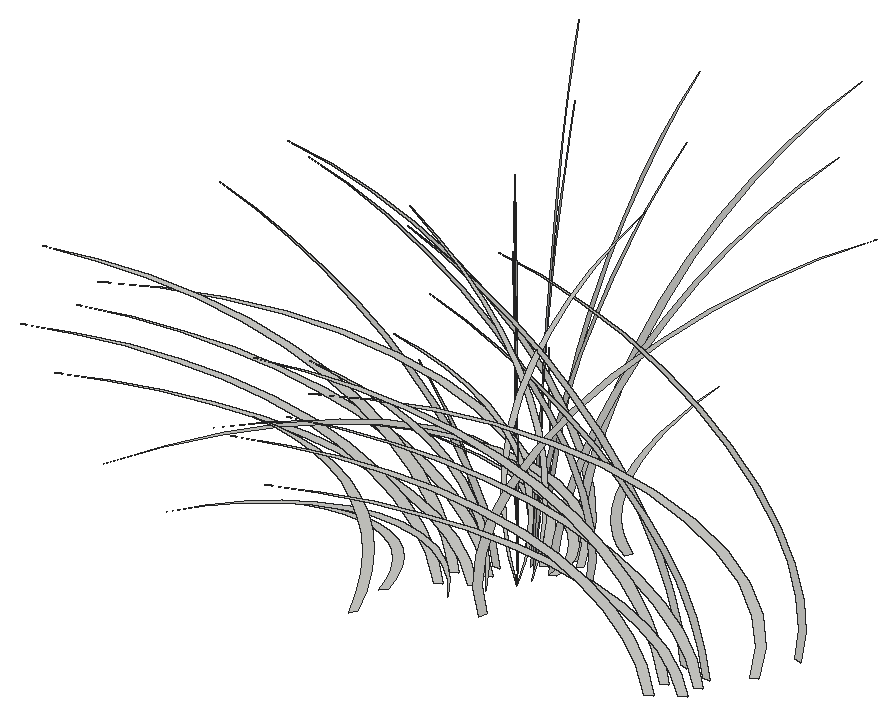
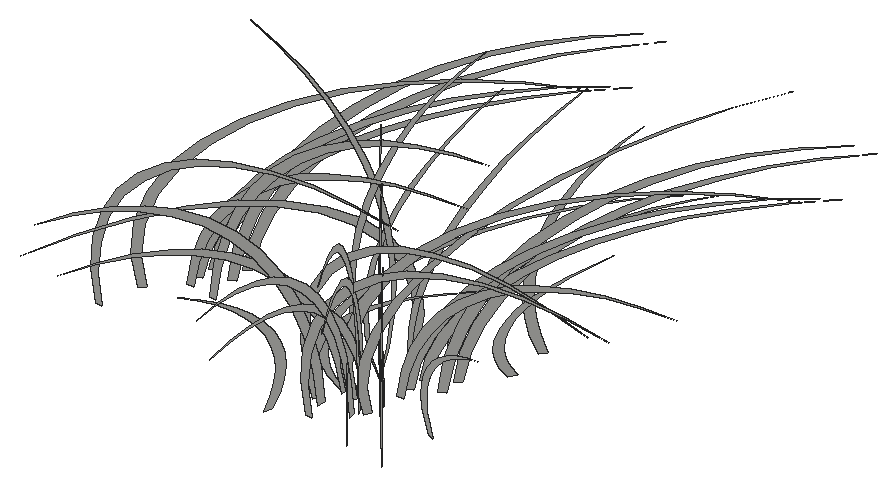
# SketchUp Ruby script. Lengths in inches.
U = 1.inch
M = Sketchup.active_model
def pt(a) = Geom::Point3d.new(a.map { |v| v * U })
def face(e, loops, mat)
  f = e.add_face(loops[0].map { |a| pt(a) })
  loops[1..].each { |l| e.add_face(l.map { |a| pt(a) }).erase! }
  f.material = f.back_material = mat if mat
  f
end
# faces: each face lists its corners as indices into pts; further lists are holes
def faces(e, pts, list, mat = nil) = list.each { |f| face(e, (f[0].is_a?(Array) ? f : [f]).map { |l| l.map { |i| pts[i] } }, mat) }
# xy, xz, yz: faces in a plane at the given z, y or x. An outline is a flat list of corners, or four numbers for a rectangle; further outlines are holes
def ring(l) = l.size == 4 ? [[l[0], l[1]], [l[2], l[1]], [l[2], l[3]], [l[0], l[3]]] : l.each_slice(2).to_a
def flat(e, list, mat, &to3) = list.each { |f| face(e, (f[0].is_a?(Array) ? f : [f]).map { |l| ring(l).map { |u, v| to3.(u, v) } }, mat) }
def xy(e, z, list, mat = nil) = flat(e, list, mat) { |x, y| [x, y, z] }
def xz(e, y, list, mat = nil) = flat(e, list, mat) { |x, z| [x, y, z] }
def yz(e, x, list, mat = nil) = flat(e, list, mat) { |y, z| [x, y, z] }
def lines(e, pts, list) = list.each { |a, b| e.add_line(pt(pts[a]), pt(pts[b])) }
# prism: a flat outline (further loops are holes) pulled along v
def prism(e, loops, v, mat = nil)
  f = face(e, loops, mat); d = Geom::Vector3d.new(v.map { |x| x * U })
  f.pushpull(f.normal.samedirection?(d) ? d.length : -d.length)
end
def box(e, o, s, mat = nil) = prism(e, [[o, [o[0] + s[0], o[1], o[2]], [o[0] + s[0], o[1] + s[1], o[2]], [o[0], o[1] + s[1], o[2]]]], [0, 0, s[2]], mat)
def at(x, y, z, deg = 0) = Geom::Transformation.translation(pt([x, y, z])) * Geom::Transformation.rotation(ORIGIN, Z_AXIS, deg.degrees)
def axes(o, x, y, z) = Geom::Transformation.new([*x, 0, *y, 0, *z, 0, *pt(o).to_a, 1])
def part(name) = M.definitions.add(name)
# library, detail: a bought-in or finely detailed component or shape, given as its bounding box
def library(name, o, s) = part(name).tap { |d| box(d.entities, o, s) }
def detail(e, o, s) = box(e.add_group.entities, o, s)
def put(e, d, t, mat = nil) = e.add_instance(d, t).tap { |i| i.material = mat if mat }
def group(e, t, mat = nil) = e.add_group.tap { |g| g.transformation = t; g.material = mat if mat }.entities
root = M.entities
p = [[75.43,134.13,1.9375],[799.67,134.13,1.9375]]
lines(root,p,[[0,1]])
g1 = group(root,at(436.95,262.29,0))
p = [[-18.45,-9.5625,18.05],[-21.23,-11,18.53],[-18.53,-9.61,17.95],[-15.93,-8.26,17.15],[-13.45,-6.97,16.14],[-11.12,-5.76,14.93],
  [-8.96,-4.64,13.53],[-7,-3.63,11.96],[-5.26,-2.73,10.23],[-3.77,-1.95,8.37],[-2.53,-1.3125,6.39],[-1.5625,-0.81,4.32],
  [-0.875,-0.45,2.18],[-0.48,-0.25,0],[0,0,0],[-0.32,-0.17,2.23],[-0.97,-0.5,4.43],[-1.92,-0.99,6.55],
  [-3.16,-1.64,8.57],[-4.69,-2.43,10.47],[-6.48,-3.36,12.22],[-8.51,-4.41,13.8],[-10.75,-5.57,15.1875],[-13.17,-6.83,16.37],
  [-15.75,-8.16,17.33]]
faces(g1,p,[[0,1,2,3,4,5,6,7,8,9,10,11,12,13,14,15,16,17,18,19,20,21,22,23,24]])
g2 = group(root,at(438.46,264.06,0))
p = [[-20.46,3.64,14.56],[-23.54,4.19,14.94],[-20.55,3.66,14.48],[-17.67,3.15,13.83],[-14.91,2.66,13.02],[-12.33,2.2,12.04],
  [-9.93,1.77,10.91],[-7.76,1.38,9.64],[-5.84,1.04,8.25],[-4.18,0.74,6.75],[-2.8,0.5,5.15],[-1.73,0.31,3.49],
  [-0.97,0.17,1.76],[-0.53,0.09,0],[0,0,0],[-0.36,0.0625,1.8],[-1.07,0.19,3.57],[-2.125,0.38,5.28],
  [-3.51,0.625,6.91],[-5.2,0.93,8.44],[-7.1875,1.28,9.85],[-9.43,1.68,11.13],[-11.92,2.125,12.25],[-14.61,2.6,13.2],
  [-17.46,3.11,13.97]]
faces(g2,p,[[0,1,2,3,4,5,6,7,8,9,10,11,12,13,14,15,16,17,18,19,20,21,22,23,24]])
g3 = group(root,at(437,260.8,0))
p = [[-17.17,-11.7,15.34],[-19.76,-13.47,15.75],[-17.25,-11.76,15.26],[-14.83,-10.11,14.58],[-12.52,-8.53,13.72],[-10.35,-7.05,12.69],
  [-8.34,-5.68,11.5],[-6.52,-4.44,10.16],[-4.9,-3.34,8.7],[-3.51,-2.39,7.11],[-2.35,-1.6,5.43],[-1.45,-0.99,3.67],
  [-0.82,-0.56,1.86],[-0.45,-0.3,0],[0,0,0],[-0.3,-0.21,1.9],[-0.9,-0.61,3.76],[-1.78,-1.22,5.57],
  [-2.95,-2.01,7.28],[-4.37,-2.98,8.9],[-6.03,-4.11,10.39],[-7.92,-5.4,11.73],[-10,-6.82,12.91],[-12.26,-8.36,13.91],
  [-14.66,-9.99,14.73]]
faces(g3,p,[[0,1,2,3,4,5,6,7,8,9,10,11,12,13,14,15,16,17,18,19,20,21,22,23,24]])
g4 = group(root,at(438.67,263.18,0))
p = [[-18.45,-9.5625,14.56],[-21.23,-11,14.94],[-18.53,-9.61,14.48],[-15.93,-8.26,13.83],[-13.45,-6.97,13.02],[-11.12,-5.76,12.04],
  [-8.96,-4.64,10.91],[-7,-3.63,9.64],[-5.26,-2.73,8.25],[-3.77,-1.95,6.75],[-2.53,-1.3125,5.15],[-1.5625,-0.81,3.49],
  [-0.875,-0.45,1.76],[-0.48,-0.25,0],[0,0,0],[-0.32,-0.17,1.8],[-0.97,-0.5,3.57],[-1.92,-0.99,5.28],
  [-3.16,-1.64,6.91],[-4.69,-2.43,8.44],[-6.48,-3.36,9.85],[-8.51,-4.41,11.13],[-10.75,-5.57,12.25],[-13.17,-6.83,13.2],
  [-15.75,-8.16,13.97]]
faces(g4,p,[[0,1,2,3,4,5,6,7,8,9,10,11,12,13,14,15,16,17,18,19,20,21,22,23,24]])
g5 = group(root,at(438.67,263.18,0))
p = [[-18.45,-9.5625,14.56],[-21.23,-11,14.94],[-18.53,-9.61,14.48],[-15.93,-8.26,13.83],[-13.45,-6.97,13.02],[-11.12,-5.76,12.04],
  [-8.96,-4.64,10.91],[-7,-3.63,9.64],[-5.26,-2.73,8.25],[-3.77,-1.95,6.75],[-2.53,-1.3125,5.15],[-1.5625,-0.81,3.49],
  [-0.875,-0.45,1.76],[-0.48,-0.25,0],[0,0,0],[-0.32,-0.17,1.8],[-0.97,-0.5,3.57],[-1.92,-0.99,5.28],
  [-3.16,-1.64,6.91],[-4.69,-2.43,8.44],[-6.48,-3.36,9.85],[-8.51,-4.41,11.13],[-10.75,-5.57,12.25],[-13.17,-6.83,13.2],
  [-15.75,-8.16,13.97]]
faces(g5,p,[[0,1,2,3,4,5,6,7,8,9,10,11,12,13,14,15,16,17,18,19,20,21,22,23,24]])
g6 = group(root,at(441.53,268.9,0))
p = [[-0.91,0.16,0],[-0.4,0.07,0],[0,0,2.0625],[-0.16,0.03,4.13],[-0.89,0.16,6.16],[-2.17,0.39,8.1],
  [-3.95,0.7,9.91],[-6.21,1.11,11.52],[-8.88,1.58,12.92],[-11.91,2.12,14.05],[-15.2,2.71,14.9],[-18.68,3.33,15.45],
  [-22.27,3.97,15.67],[-25.88,4.61,15.5625],[-22.34,3.98,15.58],[-18.84,3.36,15.29],[-15.45,2.75,14.71],[-12.26,2.18,13.83],
  [-9.34,1.66,12.68],[-6.75,1.2,11.3],[-4.56,0.8125,9.7],[-2.81,0.5,7.9375],[-1.55,0.28,6.04],[-0.8,0.14,4.05],
  [-0.59,0.1,2.02]]
faces(g6,p,[[0,1,2,3,4,5,6,7,8,9,10,11,12,13,14,15,16,17,18,19,20,21,22,23,24]])
g7 = group(root,at(441.53,268.9,0))
p = [[-0.91,0.16,0],[-0.4,0.07,0],[0,0,2.0625],[-0.16,0.03,4.13],[-0.89,0.16,6.16],[-2.17,0.39,8.1],
  [-3.95,0.7,9.91],[-6.21,1.11,11.52],[-8.88,1.58,12.92],[-11.91,2.12,14.05],[-15.2,2.71,14.9],[-18.68,3.33,15.45],
  [-22.27,3.97,15.67],[-25.88,4.61,15.5625],[-22.34,3.98,15.58],[-18.84,3.36,15.29],[-15.45,2.75,14.71],[-12.26,2.18,13.83],
  [-9.34,1.66,12.68],[-6.75,1.2,11.3],[-4.56,0.8125,9.7],[-2.81,0.5,7.9375],[-1.55,0.28,6.04],[-0.8,0.14,4.05],
  [-0.59,0.1,2.02]]
faces(g7,p,[[0,1,2,3,4,5,6,7,8,9,10,11,12,13,14,15,16,17,18,19,20,21,22,23,24]])
g8 = group(root,at(438.59,261.89,0))
p = [[-17.17,-11.7,12.375],[-19.76,-13.47,12.7],[-17.25,-11.76,12.31],[-14.83,-10.11,11.76],[-12.52,-8.53,11.07],[-10.35,-7.05,10.23],
  [-8.34,-5.68,9.27],[-6.52,-4.44,8.2],[-4.9,-3.34,7.01],[-3.51,-2.39,5.74],[-2.35,-1.6,4.38],[-1.45,-0.99,2.96],
  [-0.82,-0.56,1.5],[-0.45,-0.3,0],[0,0,0],[-0.3,-0.21,1.53],[-0.9,-0.61,3.03],[-1.78,-1.22,4.49],
  [-2.95,-2.01,5.875],[-4.37,-2.98,7.18],[-6.03,-4.11,8.375],[-7.92,-5.4,9.46],[-10,-6.82,10.41],[-12.26,-8.36,11.22],
  [-14.66,-9.99,11.88]]
faces(g8,p,[[0,1,2,3,4,5,6,7,8,9,10,11,12,13,14,15,16,17,18,19,20,21,22,23,24]])
g9 = group(root,at(440.79,266.21,0))
p = [[-0.82,-0.43,0],[-0.36,-0.1875,0],[0,0,2.0625],[-0.15,-0.08,4.13],[-0.8,-0.42,6.16],[-1.95,-1.01,8.1],
  [-3.57,-1.85,9.91],[-5.6,-2.9,11.52],[-8.01,-4.15,12.92],[-10.74,-5.57,14.05],[-13.71,-7.1,14.9],[-16.85,-8.73,15.45],
  [-20.09,-10.41,15.67],[-23.34,-12.1,15.5625],[-20.15,-10.44,15.58],[-16.99,-8.81,15.29],[-13.9375,-7.22,14.71],[-11.06,-5.73,13.83],
  [-8.42,-4.37,12.68],[-6.09,-3.16,11.3],[-4.11,-2.13,9.7],[-2.53,-1.3125,7.9375],[-1.4,-0.72,6.04],[-0.72,-0.375,4.05],
  [-0.53,-0.27,2.02]]
faces(g9,p,[[0,1,2,3,4,5,6,7,8,9,10,11,12,13,14,15,16,17,18,19,20,21,22,23,24]])
g10 = group(root,at(444.39,265.34,0))
p = [[-0.95,0.28,0],[-0.42,0.125,0],[0,0,2.01],[-0.17,0.05,4.04],[-0.93,0.27,6.02],[-2.27,0.66,7.92],
  [-4.14,1.21,9.68],[-6.5,1.9,11.26],[-9.3,2.72,12.62],[-12.46,3.64,13.73],[-15.91,4.65,14.5625],[-19.55,5.72,15.09],
  [-23.3125,6.82,15.31],[-27.08,7.92,15.2],[-23.38,6.84,15.22],[-19.72,5.77,14.94],[-16.17,4.73,14.37],[-12.83,3.75,13.51],
  [-9.77,2.86,12.39],[-7.0625,2.07,11.04],[-4.77,1.39,9.48],[-2.94,0.86,7.75],[-1.62,0.47,5.9],[-0.84,0.25,3.96],
  [-0.61,0.18,1.98]]
faces(g10,p,[[0,1,2,3,4,5,6,7,8,9,10,11,12,13,14,15,16,17,18,19,20,21,22,23,24]])
g11 = group(root,at(435.12,266.09,0))
p = [[-6.53,2.99,7.88],[-5.33,2.44,7.38],[-4.26,1.95,6.83],[-3.3,1.51,6.24],[-2.48,1.14,5.62],[-1.81,0.83,4.96],
  [-1.28,0.58,4.27],[-0.9,0.41,3.57],[-0.68,0.31,2.86],[-0.61,0.28,2.13],[-0.71,0.32,1.41],[-0.96,0.4375,0.7],
  [-1.37,0.625,0],[-0.84,0.38,0],[-0.39,0.18,0.71],[-0.11,0.05,1.43],[0,0,2.17],[-0.07,0.03,2.9],
  [-0.32,0.15,3.63],[-0.74,0.34,4.34],[-1.33,0.61,5.03],[-2.08,0.95,5.69],[-2.99,1.37,6.3125],[-4.04,1.85,6.89],
  [-5.22,2.39,7.41]]
faces(g11,p,[[0,1,2,3,4,5,6,7,8,9,10,11,12,13,14,15,16,17,18,19,20,21,22,23,24]])
g12 = group(root,at(437.88,266.32,0))
p = [[-10.66,12.98,9.9],[-9.23,11.23,9.83],[-7.82,9.52,9.59],[-6.46,7.86,9.18],[-5.18,6.3,8.61],[-3.99,4.86,7.88],
  [-2.93,3.57,7.02],[-2.02,2.46,6.03],[-1.27,1.54,4.95],[-0.6875,0.84,3.78],[-0.29,0.36,2.55],[-0.1,0.12,1.28],
  [-0.09,0.12,0],[0,0,1.3],[-0.125,0.15,2.61],[-0.47,0.57,3.875],[-1.02,1.24,5.09],[-1.77,2.15,6.21],
  [-2.69,3.28,7.22],[-3.78,4.6,8.1],[-5,6.09,8.82],[-6.33,7.71,9.37],[-7.74,9.43,9.74],[-9.2,11.19,9.92]]
faces(g12,p,[[0,1,2,3,4,5,6,7,8,9,10,11,12,13,14,15,16,17,18,19,20,21,22,23]])
g13 = group(root,at(439.14,266.59,0))
p = [[-11.32,17.43,20.75],[-13.02,20.05,21.3],[-11.37,17.51,20.63],[-9.77,15.05,19.72],[-8.25,12.7,18.55],[-6.82,10.5,17.16],
  [-5.5,8.46,15.55],[-4.29,6.61,13.74],[-3.23,4.97,11.76],[-2.3125,3.56,9.62],[-1.55,2.39,7.35],[-0.96,1.47,4.97],
  [-0.54,0.83,2.51],[-0.29,0.45,0],[0,0,0],[-0.2,0.31,2.57],[-0.59,0.91,5.09],[-1.18,1.8125,7.53],
  [-1.94,2.99,9.85],[-2.88,4.43,12.03],[-3.98,6.12,14.04],[-5.22,8.04,15.86],[-6.59,10.15,17.46],[-8.08,12.44,18.82],
  [-9.66,14.88,19.92]]
faces(g13,p,[[0,1,2,3,4,5,6,7,8,9,10,11,12,13,14,15,16,17,18,19,20,21,22,23,24]])
g14 = group(root,at(435.02,269.81,0))
p = [[-4.56,5.55,16.02],[-3.72,4.53,15.01],[-2.97,3.62,13.89],[-2.31,2.81,12.69],[-1.73,2.11,11.42],[-1.26,1.54,10.08],
  [-0.89,1.09,8.6875],[-0.63,0.76,7.26],[-0.47,0.58,5.8],[-0.43,0.52,4.34],[-0.49,0.6,2.87],[-0.67,0.81,1.42],
  [-0.95,1.16,0],[-0.59,0.71,0],[-0.27,0.33,1.44],[-0.07,0.09,2.92],[0,0,4.41],[-0.05,0.0625,5.9],
  [-0.22,0.27,7.38],[-0.52,0.63,8.83],[-0.93,1.13,10.23],[-1.45,1.77,11.57],[-2.09,2.54,12.83],[-2.82,3.43,14.01],
  [-3.65,4.44,15.07]]
faces(g14,p,[[0,1,2,3,4,5,6,7,8,9,10,11,12,13,14,15,16,17,18,19,20,21,22,23,24]])
g15 = group(root,at(435.02,269.81,0))
p = [[-4.56,5.55,16.02],[-3.72,4.53,15.01],[-2.97,3.62,13.89],[-2.31,2.81,12.69],[-1.73,2.11,11.42],[-1.26,1.54,10.08],
  [-0.89,1.09,8.6875],[-0.63,0.76,7.26],[-0.47,0.58,5.8],[-0.43,0.52,4.34],[-0.49,0.6,2.87],[-0.67,0.81,1.42],
  [-0.95,1.16,0],[-0.59,0.71,0],[-0.27,0.33,1.44],[-0.07,0.09,2.92],[0,0,4.41],[-0.05,0.0625,5.9],
  [-0.22,0.27,7.38],[-0.52,0.63,8.83],[-0.93,1.13,10.23],[-1.45,1.77,11.57],[-2.09,2.54,12.83],[-2.82,3.43,14.01],
  [-3.65,4.44,15.07]]
faces(g15,p,[[0,1,2,3,4,5,6,7,8,9,10,11,12,13,14,15,16,17,18,19,20,21,22,23,24]])
g16 = group(root,at(438.71,267.4,0))
p = [[-0.37,-0.92,0],[-0.16,-0.41,0],[0,0,1.75],[-0.07,-0.17,3.51],[-0.36,-0.9,5.24],[-0.88,-2.19,6.89],
  [-1.61,-4,8.42],[-2.53,-6.28,9.8],[-3.61,-8.99,10.98],[-4.84,-12.04,11.95],[-6.18,-15.375,12.67],[-7.6,-18.9,13.13],
  [-9.06,-22.53,13.32],[-10.53,-26.18,13.23],[-9.09,-22.6,13.25],[-7.66,-19.06,13],[-6.29,-15.63,12.5],[-4.99,-12.41,11.75],
  [-3.8,-9.45,10.78],[-2.75,-6.83,9.6],[-1.85,-4.61,8.25],[-1.14,-2.84,6.75],[-0.63,-1.57,5.13],[-0.33,-0.8125,3.44],
  [-0.24,-0.59,1.72]]
faces(g16,p,[[0,1,2,3,4,5,6,7,8,9,10,11,12,13,14,15,16,17,18,19,20,21,22,23,24]])
g17 = group(root,at(435.45,259.21,0))
p = [[-3.94,-6,6.7],[-3.22,-4.9,6.27],[-2.57,-3.91,5.81],[-2,-3.04,5.31],[-1.5,-2.28,4.77],[-1.09,-1.66,4.21],
  [-0.77,-1.17,3.63],[-0.54,-0.83,3.03],[-0.41,-0.62,2.43],[-0.37,-0.5625,1.8125],[-0.43,-0.65,1.2],[-0.58,-0.88,0.59],
  [-0.83,-1.26,0],[-0.51,-0.77,0],[-0.23,-0.36,0.6],[-0.0625,-0.1,1.22],[0,0,1.84],[-0.04,-0.07,2.47],
  [-0.19,-0.29,3.09],[-0.45,-0.68,3.69],[-0.8,-1.22,4.28],[-1.26,-1.91,4.84],[-1.81,-2.75,5.37],[-2.44,-3.71,5.86],
  [-3.16,-4.8,6.3]]
faces(g17,p,[[0,1,2,3,4,5,6,7,8,9,10,11,12,13,14,15,16,17,18,19,20,21,22,23,24]])
g18 = group(root,at(438.22,259.91,0))
p = [[-9.23,-14.04,8.41],[-7.99,-12.15,8.36],[-6.77,-10.29,8.15],[-5.59,-8.5,7.8],[-4.48,-6.8125,7.32],[-3.46,-5.26,6.7],
  [-2.54,-3.86,5.97],[-1.75,-2.66,5.13],[-1.09,-1.67,4.2],[-0.59,-0.9,3.21],[-0.25,-0.39,2.16],[-0.08,-0.125,1.09],
  [-0.08,-0.125,0],[0,0,1.11],[-0.11,-0.16,2.21],[-0.4,-0.61,3.29],[-0.88,-1.34,4.32],[-1.53,-2.33,5.28],
  [-2.33,-3.55,6.14],[-3.27,-4.98,6.88],[-4.33,-6.59,7.5],[-5.48,-8.34,7.97],[-6.7,-10.19,8.28],[-7.96,-12.11,8.43]]
faces(g18,p,[[0,1,2,3,4,5,6,7,8,9,10,11,12,13,14,15,16,17,18,19,20,21,22,23]])
g19 = group(root,at(440.1875,264.97,0))
p = [[-11.32,17.43,16.73],[-13.02,20.05,17.17],[-11.37,17.51,16.64],[-9.77,15.05,15.9],[-8.25,12.7,14.96],[-6.82,10.5,13.84],
  [-5.5,8.46,12.54],[-4.29,6.61,11.08],[-3.23,4.97,9.48],[-2.3125,3.56,7.76],[-1.55,2.39,5.92],[-0.96,1.47,4.01],
  [-0.54,0.83,2.02],[-0.29,0.45,0],[0,0,0],[-0.2,0.31,2.07],[-0.59,0.91,4.1],[-1.18,1.8125,6.07],
  [-1.94,2.99,7.94],[-2.88,4.43,9.7],[-3.98,6.12,11.33],[-5.22,8.04,12.79],[-6.59,10.15,14.08],[-8.08,12.44,15.17],
  [-9.66,14.88,16.0625]]
faces(g19,p,[[0,1,2,3,4,5,6,7,8,9,10,11,12,13,14,15,16,17,18,19,20,21,22,23,24]])
g20 = group(root,at(435.74,256.13,0))
p = [[-3.94,-6,13.62],[-3.22,-4.9,12.76],[-2.57,-3.91,11.81],[-2,-3.04,10.79],[-1.5,-2.28,9.7],[-1.09,-1.66,8.57],
  [-0.77,-1.17,7.38],[-0.54,-0.83,6.17],[-0.41,-0.62,4.93],[-0.37,-0.5625,3.6875],[-0.43,-0.65,2.44],[-0.58,-0.88,1.21],
  [-0.83,-1.26,0],[-0.51,-0.77,0],[-0.23,-0.36,1.22],[-0.0625,-0.1,2.48],[0,0,3.75],[-0.04,-0.07,5.02],
  [-0.19,-0.29,6.28],[-0.45,-0.68,7.51],[-0.8,-1.22,8.7],[-1.26,-1.91,9.84],[-1.81,-2.75,10.91],[-2.44,-3.71,11.9],
  [-3.16,-4.8,12.8125]]
faces(g20,p,[[0,1,2,3,4,5,6,7,8,9,10,11,12,13,14,15,16,17,18,19,20,21,22,23,24]])
g21 = group(root,at(442.21,267.55,0))
p = [[-0.5,-0.57,0],[-0.22,-0.25,0],[0,0,1.46],[-0.09,-0.1,2.93],[-0.49,-0.56,4.375],[-1.19,-1.35,5.75],
  [-2.17,-2.47,7.03],[-3.41,-3.89,8.18],[-4.88,-5.56,9.17],[-6.54,-7.45,9.98],[-8.36,-9.51,10.58],[-10.27,-11.69,10.97],
  [-12.24,-13.9375,11.125],[-14.23,-16.19,11.05],[-12.28,-13.98,11.0625],[-10.36,-11.79,10.86],[-8.5,-9.67,10.44],[-6.74,-7.67,9.82],
  [-5.13,-5.84,9.01],[-3.71,-4.22,8.02],[-2.51,-2.85,6.89],[-1.54,-1.76,5.64],[-0.85,-0.97,4.29],[-0.44,-0.5,2.88],
  [-0.32,-0.37,1.4375]]
faces(g21,p,[[0,1,2,3,4,5,6,7,8,9,10,11,12,13,14,15,16,17,18,19,20,21,22,23,24]])
g22 = group(root,at(442.21,267.55,0))
p = [[-0.5,-0.57,0],[-0.22,-0.25,0],[0,0,1.46],[-0.09,-0.1,2.93],[-0.49,-0.56,4.375],[-1.19,-1.35,5.75],
  [-2.17,-2.47,7.03],[-3.41,-3.89,8.18],[-4.88,-5.56,9.17],[-6.54,-7.45,9.98],[-8.36,-9.51,10.58],[-10.27,-11.69,10.97],
  [-12.24,-13.9375,11.125],[-14.23,-16.19,11.05],[-12.28,-13.98,11.0625],[-10.36,-11.79,10.86],[-8.5,-9.67,10.44],[-6.74,-7.67,9.82],
  [-5.13,-5.84,9.01],[-3.71,-4.22,8.02],[-2.51,-2.85,6.89],[-1.54,-1.76,5.64],[-0.85,-0.97,4.29],[-0.44,-0.5,2.88],
  [-0.32,-0.37,1.4375]]
faces(g22,p,[[0,1,2,3,4,5,6,7,8,9,10,11,12,13,14,15,16,17,18,19,20,21,22,23,24]])
g23 = group(root,at(439.1,267.22,0))
p = [[-6.07,19.87,18.05],[-6.99,22.87,18.53],[-6.1,19.96,17.95],[-5.25,17.16,17.15],[-4.43,14.49,16.14],[-3.66,11.97,14.93],
  [-2.95,9.65,13.53],[-2.31,7.54,11.96],[-1.73,5.67,10.23],[-1.24,4.06,8.37],[-0.83,2.72,6.39],[-0.51,1.68,4.32],
  [-0.29,0.94,2.18],[-0.16,0.52,0],[0,0,0],[-0.11,0.35,2.23],[-0.32,1.04,4.43],[-0.63,2.07,6.55],
  [-1.04,3.41,8.57],[-1.55,5.05,10.47],[-2.13,6.98,12.22],[-2.8,9.16,13.8],[-3.54,11.58,15.1875],[-4.34,14.1875,16.37],
  [-5.1875,16.96,17.33]]
faces(g23,p,[[0,1,2,3,4,5,6,7,8,9,10,11,12,13,14,15,16,17,18,19,20,21,22,23,24]])
g24 = group(root,at(438.04,269.17,0))
p = [[-4.56,5.55,7.88],[-3.72,4.53,7.38],[-2.97,3.62,6.83],[-2.31,2.81,6.24],[-1.73,2.11,5.62],[-1.26,1.54,4.96],
  [-0.89,1.09,4.27],[-0.63,0.76,3.57],[-0.47,0.58,2.86],[-0.43,0.52,2.13],[-0.49,0.6,1.41],[-0.67,0.81,0.7],
  [-0.95,1.16,0],[-0.59,0.71,0],[-0.27,0.33,0.71],[-0.07,0.09,1.43],[0,0,2.17],[-0.05,0.0625,2.9],
  [-0.22,0.27,3.63],[-0.52,0.63,4.34],[-0.93,1.13,5.03],[-1.45,1.77,5.69],[-2.09,2.54,6.3125],[-2.82,3.43,6.89],
  [-3.65,4.44,7.41]]
faces(g24,p,[[0,1,2,3,4,5,6,7,8,9,10,11,12,13,14,15,16,17,18,19,20,21,22,23,24]])
g25 = group(root,at(439.33,264.5625,0))
p = [[-6.74,8.21,19.61],[-5.67,6.9,18.16],[-4.68,5.7,16.67],[-3.78,4.6,15.125],[-2.98,3.62,13.55],[-2.27,2.76,11.93],
  [-1.65,2.01,10.28],[-1.14,1.39,8.61],[-0.72,0.88,6.91],[-0.41,0.5,5.2],[-0.2,0.24,3.47],[-0.09,0.11,1.74],
  [-0.09,0.11,0],[0,0,1.74],[-0.03,0.04,3.49],[-0.1875,0.23,5.23],[-0.46,0.56,6.96],[-0.85,1.04,8.67],
  [-1.36,1.66,10.36],[-1.98,2.42,12.01],[-2.72,3.3125,13.63],[-3.57,4.35,15.21],[-4.52,5.51,16.73],[-5.58,6.8,18.2]]
faces(g25,p,[[0,1,2,3,4,5,6,7,8,9,10,11,12,13,14,15,16,17,18,19,20,21,22,23]])
g26 = group(root,at(439.33,264.5625,0))
p = [[-6.74,8.21,19.61],[-5.67,6.9,18.16],[-4.68,5.7,16.67],[-3.78,4.6,15.125],[-2.98,3.62,13.55],[-2.27,2.76,11.93],
  [-1.65,2.01,10.28],[-1.14,1.39,8.61],[-0.72,0.88,6.91],[-0.41,0.5,5.2],[-0.2,0.24,3.47],[-0.09,0.11,1.74],
  [-0.09,0.11,0],[0,0,1.74],[-0.03,0.04,3.49],[-0.1875,0.23,5.23],[-0.46,0.56,6.96],[-0.85,1.04,8.67],
  [-1.36,1.66,10.36],[-1.98,2.42,12.01],[-2.72,3.3125,13.63],[-3.57,4.35,15.21],[-4.52,5.51,16.73],[-5.58,6.8,18.2]]
faces(g26,p,[[0,1,2,3,4,5,6,7,8,9,10,11,12,13,14,15,16,17,18,19,20,21,22,23]])
g27 = group(root,at(439.67,265.375,0))
p = [[-6.07,19.87,14.56],[-6.99,22.87,14.94],[-6.1,19.96,14.48],[-5.25,17.16,13.83],[-4.43,14.49,13.02],[-3.66,11.97,12.04],
  [-2.95,9.65,10.91],[-2.31,7.54,9.64],[-1.73,5.67,8.25],[-1.24,4.06,6.75],[-0.83,2.72,5.15],[-0.51,1.68,3.49],
  [-0.29,0.94,1.76],[-0.16,0.52,0],[0,0,0],[-0.11,0.35,1.8],[-0.32,1.04,3.57],[-0.63,2.07,5.28],
  [-1.04,3.41,6.91],[-1.55,5.05,8.44],[-2.13,6.98,9.85],[-2.8,9.16,11.13],[-3.54,11.58,12.25],[-4.34,14.1875,13.2],
  [-5.1875,16.96,13.97]]
faces(g27,p,[[0,1,2,3,4,5,6,7,8,9,10,11,12,13,14,15,16,17,18,19,20,21,22,23,24]])
g28 = group(root,at(439.47,261.81,0))
p = [[-5.83,-8.875,16.67],[-4.9,-7.46,15.44],[-4.05,-6.16,14.17],[-3.27,-4.98,12.86],[-2.58,-3.92,11.51],[-1.96,-2.98,10.14],
  [-1.43,-2.18,8.74],[-0.99,-1.5,7.31],[-0.63,-0.95,5.87],[-0.36,-0.54,4.42],[-0.17,-0.26,2.95],[-0.08,-0.12,1.48],
  [-0.08,-0.12,0],[0,0,1.48],[-0.03,-0.04,2.97],[-0.16,-0.24,4.45],[-0.4,-0.6,5.92],[-0.74,-1.12,7.37],
  [-1.18,-1.79,8.81],[-1.72,-2.61,10.21],[-2.36,-3.58,11.59],[-3.09,-4.7,12.93],[-3.92,-5.96,14.22],[-4.83,-7.35,15.47]]
faces(g28,p,[[0,1,2,3,4,5,6,7,8,9,10,11,12,13,14,15,16,17,18,19,20,21,22,23]])
g29 = group(root,at(441.58,264.53,0))
p = [[-0.89,-0.32,0],[-0.4,-0.14,1.97],[-0.1,-0.04,3.96],[0,0,5.95],[-0.1,-0.03,7.95],[-0.39,-0.14,9.9375],
  [-0.89,-0.3125,11.91],[-1.57,-0.56,13.85],[-2.45,-0.87,15.76],[-3.52,-1.25,17.63],[-4.77,-1.6875,19.44],[-6.19,-2.19,21.2],
  [-7.79,-2.76,22.89],[-6.29,-2.23,21.17],[-4.94,-1.75,19.4],[-3.76,-1.33,17.58],[-2.74,-0.97,15.71],[-1.89,-0.67,13.8],
  [-1.22,-0.43,11.86],[-0.72,-0.25,9.9],[-0.4,-0.14,7.93],[-0.25,-0.09,5.94],[-0.29,-0.1,3.95],[-0.5,-0.18,1.97]]
faces(g29,p,[[0,1,2,3,4,5,6,7,8,9,10,11,12,13,14,15,16,17,18,19,20,21,22,23]])
g30 = group(root,at(442.68,265.89,0))
p = [[-9.01,-2.98,7.88],[-7.3,-2.41,7.38],[-5.75,-1.9,6.83],[-4.38,-1.45,6.24],[-3.2,-1.06,5.62],[-2.23,-0.74,4.96],
  [-1.47,-0.49,4.27],[-0.92,-0.31,3.57],[-0.61,-0.2,2.86],[-0.51,-0.17,2.13],[-0.65,-0.21,1.41],[-1.01,-0.33,0.7],
  [-1.6,-0.53,0],[-1.21,-0.4,0],[-0.54,-0.18,0.69],[-0.12,-0.04,1.4],[0.06,0.02,2.13],[-0.02,-0.01,2.85],
  [-0.35,-0.11,3.58],[-0.92,-0.3,4.29],[-1.73,-0.57,4.98],[-2.78,-0.92,5.64],[-4.05,-1.34,6.27],[-5.52,-1.82,6.86],
  [-7.18,-2.375,7.4]]
faces(g30,p,[[0,1,2,3,4,5,6,7,8,9,10,11,12,13,14,15,16,17,18,19,20,21,22,23,24]])
g31 = group(root,at(441.01,262.51,0))
p = [[-0.6,0.73,0],[-0.27,0.33,1.77],[-0.07,0.08,3.57],[0,0,5.36],[-0.07,0.08,7.16],[-0.27,0.32,8.95],
  [-0.6,0.73,10.73],[-1.06,1.29,12.48],[-1.65,2.01,14.2],[-2.37,2.88,15.88],[-3.21,3.91,17.52],[-4.17,5.08,19.1],
  [-5.25,6.39,20.625],[-4.23,5.15,19.08],[-3.33,4.05,17.48],[-2.53,3.08,15.83],[-1.84,2.25,14.15],[-1.27,1.55,12.43],
  [-0.82,1,10.6875],[-0.48,0.59,8.92],[-0.27,0.32,7.14],[-0.17,0.21,5.35],[-0.19,0.24,3.5625],[-0.34,0.41,1.78]]
faces(g31,p,[[0,1,2,3,4,5,6,7,8,9,10,11,12,13,14,15,16,17,18,19,20,21,22,23]])
g32 = group(root,at(440.93,264.03,0))
p = [[-0.52,-0.79,0],[-0.23,-0.35,1.51],[-0.06,-0.09,3.03],[0,0,4.56],[-0.06,-0.09,6.09],[-0.23,-0.35,7.61],
  [-0.52,-0.79,9.12],[-0.92,-1.39,10.61],[-1.43,-2.17,12.07],[-2.05,-3.12,13.5],[-2.78,-4.23,14.89],[-3.61,-5.49,16.24],
  [-4.54,-6.91,17.53],[-3.66,-5.57,16.21],[-2.88,-4.38,14.86],[-2.1875,-3.33,13.46],[-1.6,-2.43,12.03],[-1.1,-1.68,10.57],
  [-0.71,-1.08,9.08],[-0.42,-0.64,7.58],[-0.23,-0.35,6.07],[-0.15,-0.22,4.55],[-0.17,-0.25,3.03],[-0.29,-0.44,1.51]]
faces(g32,p,[[0,1,2,3,4,5,6,7,8,9,10,11,12,13,14,15,16,17,18,19,20,21,22,23]])
g33 = group(root,at(441.04,265.26,0))
p = [[1.63,20.71,16.73],[1.875,23.84,17.17],[1.64,20.8125,16.64],[1.41,17.89,15.9],[1.1875,15.1,14.96],[0.98,12.48,13.84],
  [0.79,10.06,12.54],[0.62,7.86,11.08],[0.47,5.91,9.48],[0.33,4.23,7.76],[0.22,2.84,5.92],[0.14,1.75,4.01],
  [0.08,0.98,2.02],[0.04,0.54,0],[0,0,0],[0.03,0.36,2.07],[0.09,1.09,4.1],[0.17,2.15,6.07],
  [0.28,3.55,7.94],[0.41,5.27,9.7],[0.57,7.28,11.33],[0.75,9.55,12.79],[0.95,12.07,14.08],[1.16,14.79,15.17],
  [1.39,17.68,16.0625]]
faces(g33,p,[[0,1,2,3,4,5,6,7,8,9,10,11,12,13,14,15,16,17,18,19,20,21,22,23,24]])
g34 = group(root,at(453.87,261.74,0))
p = [[-20.46,3.64,18.05],[-23.54,4.19,18.53],[-20.55,3.66,17.95],[-17.67,3.15,17.15],[-14.91,2.66,16.14],[-12.33,2.2,14.93],
  [-9.93,1.77,13.53],[-7.76,1.38,11.96],[-5.84,1.04,10.23],[-4.18,0.74,8.37],[-2.8,0.5,6.39],[-1.73,0.31,4.32],
  [-0.97,0.17,2.18],[-0.53,0.09,0],[0,0,0],[-0.36,0.0625,2.23],[-1.07,0.19,4.43],[-2.125,0.38,6.55],
  [-3.51,0.625,8.57],[-5.2,0.93,10.47],[-7.1875,1.28,12.22],[-9.43,1.68,13.8],[-11.92,2.125,15.1875],[-14.61,2.6,16.37],
  [-17.46,3.11,17.33]]
faces(g34,p,[[0,1,2,3,4,5,6,7,8,9,10,11,12,13,14,15,16,17,18,19,20,21,22,23,24]])
g35 = group(root,at(441.1875,267.19,0))
p = [[1.63,20.71,20.75],[1.875,23.84,21.3],[1.64,20.8125,20.63],[1.41,17.89,19.72],[1.1875,15.1,18.55],[0.98,12.48,17.16],
  [0.79,10.06,15.55],[0.62,7.86,13.74],[0.47,5.91,11.76],[0.33,4.23,9.62],[0.22,2.84,7.35],[0.14,1.75,4.97],
  [0.08,0.98,2.51],[0.04,0.54,0],[0,0,0],[0.03,0.36,2.57],[0.09,1.09,5.09],[0.17,2.15,7.53],
  [0.28,3.55,9.85],[0.41,5.27,12.03],[0.57,7.28,14.04],[0.75,9.55,15.86],[0.95,12.07,17.46],[1.16,14.79,18.82],
  [1.39,17.68,19.92]]
faces(g35,p,[[0,1,2,3,4,5,6,7,8,9,10,11,12,13,14,15,16,17,18,19,20,21,22,23,24]])
g36 = group(root,at(439.74,262.57,0))
p = [[0.67,0.67,0],[0.3,0.3,2.04],[0.08,0.08,4.1],[0,0,6.17],[0.07,0.07,8.23],[0.3,0.3,10.29],
  [0.66,0.66,12.33],[1.18,1.18,14.34],[1.84,1.84,16.32],[2.64,2.64,18.26],[3.58,3.58,20.14],[4.65,4.65,21.96],
  [5.84,5.84,23.71],[4.72,4.72,21.93],[3.71,3.71,20.09],[2.82,2.82,18.2],[2.05,2.05,16.26],[1.42,1.42,14.29],
  [0.91,0.91,12.29],[0.54,0.54,10.26],[0.3,0.3,8.21],[0.1875,0.1875,6.15],[0.22,0.22,4.09],[0.375,0.375,2.04]]
faces(g36,p,[[0,1,2,3,4,5,6,7,8,9,10,11,12,13,14,15,16,17,18,19,20,21,22,23]])
g37 = group(root,at(454.26,259.64,0))
p = [[-18.45,-9.5625,18.05],[-21.23,-11,18.53],[-18.53,-9.61,17.95],[-15.93,-8.26,17.15],[-13.45,-6.97,16.14],[-11.12,-5.76,14.93],
  [-8.96,-4.64,13.53],[-7,-3.63,11.96],[-5.26,-2.73,10.23],[-3.77,-1.95,8.37],[-2.53,-1.3125,6.39],[-1.5625,-0.81,4.32],
  [-0.875,-0.45,2.18],[-0.48,-0.25,0],[0,0,0],[-0.32,-0.17,2.23],[-0.97,-0.5,4.43],[-1.92,-0.99,6.55],
  [-3.16,-1.64,8.57],[-4.69,-2.43,10.47],[-6.48,-3.36,12.22],[-8.51,-4.41,13.8],[-10.75,-5.57,15.1875],[-13.17,-6.83,16.37],
  [-15.75,-8.16,17.33]]
faces(g37,p,[[0,1,2,3,4,5,6,7,8,9,10,11,12,13,14,15,16,17,18,19,20,21,22,23,24]])
g38 = group(root,at(454.26,259.64,0))
p = [[-18.45,-9.5625,18.05],[-21.23,-11,18.53],[-18.53,-9.61,17.95],[-15.93,-8.26,17.15],[-13.45,-6.97,16.14],[-11.12,-5.76,14.93],
  [-8.96,-4.64,13.53],[-7,-3.63,11.96],[-5.26,-2.73,10.23],[-3.77,-1.95,8.37],[-2.53,-1.3125,6.39],[-1.5625,-0.81,4.32],
  [-0.875,-0.45,2.18],[-0.48,-0.25,0],[0,0,0],[-0.32,-0.17,2.23],[-0.97,-0.5,4.43],[-1.92,-0.99,6.55],
  [-3.16,-1.64,8.57],[-4.69,-2.43,10.47],[-6.48,-3.36,12.22],[-8.51,-4.41,13.8],[-10.75,-5.57,15.1875],[-13.17,-6.83,16.37],
  [-15.75,-8.16,17.33]]
faces(g38,p,[[0,1,2,3,4,5,6,7,8,9,10,11,12,13,14,15,16,17,18,19,20,21,22,23,24]])
g39 = group(root,at(442.73,268.78,0))
p = [[2.34,6.79,9.0625],[1.91,5.55,8.49],[1.52,4.43,7.85],[1.18,3.44,7.18],[0.89,2.58,6.45],[0.65,1.88,5.7],
  [0.46,1.33,4.91],[0.32,0.93,4.1],[0.24,0.7,3.28],[0.22,0.64,2.45],[0.25,0.74,1.625],[0.34,1,0.8],
  [0.49,1.42,0],[0.3,0.875,0],[0.14,0.4,0.81],[0.04,0.11,1.65],[0,0,2.49],[0.03,0.07,3.34],
  [0.11,0.33,4.17],[0.27,0.77,4.99],[0.48,1.38,5.79],[0.75,2.17,6.54],[1.07,3.11,7.26],[1.45,4.2,7.92],
  [1.87,5.43,8.52]]
faces(g39,p,[[0,1,2,3,4,5,6,7,8,9,10,11,12,13,14,15,16,17,18,19,20,21,22,23,24]])
g40 = group(root,at(455.77,261.4,0))
p = [[-20.46,3.64,14.56],[-23.54,4.19,14.94],[-20.55,3.66,14.48],[-17.67,3.15,13.83],[-14.91,2.66,13.02],[-12.33,2.2,12.04],
  [-9.93,1.77,10.91],[-7.76,1.38,9.64],[-5.84,1.04,8.25],[-4.18,0.74,6.75],[-2.8,0.5,5.15],[-1.73,0.31,3.49],
  [-0.97,0.17,1.76],[-0.53,0.09,0],[0,0,0],[-0.36,0.0625,1.8],[-1.07,0.19,3.57],[-2.125,0.38,5.28],
  [-3.51,0.625,6.91],[-5.2,0.93,8.44],[-7.1875,1.28,9.85],[-9.43,1.68,11.13],[-11.92,2.125,12.25],[-14.61,2.6,13.2],
  [-17.46,3.11,13.97]]
faces(g40,p,[[0,1,2,3,4,5,6,7,8,9,10,11,12,13,14,15,16,17,18,19,20,21,22,23,24]])
g41 = group(root,at(454.31,258.15,0))
p = [[-17.17,-11.7,15.34],[-19.76,-13.47,15.75],[-17.25,-11.76,15.26],[-14.83,-10.11,14.58],[-12.52,-8.53,13.72],[-10.35,-7.05,12.69],
  [-8.34,-5.68,11.5],[-6.52,-4.44,10.16],[-4.9,-3.34,8.7],[-3.51,-2.39,7.11],[-2.35,-1.6,5.43],[-1.45,-0.99,3.67],
  [-0.82,-0.56,1.86],[-0.45,-0.3,0],[0,0,0],[-0.3,-0.21,1.9],[-0.9,-0.61,3.76],[-1.78,-1.22,5.57],
  [-2.95,-2.01,7.28],[-4.37,-2.98,8.9],[-6.03,-4.11,10.39],[-7.92,-5.4,11.73],[-10,-6.82,12.91],[-12.26,-8.36,13.91],
  [-14.66,-9.99,14.73]]
faces(g41,p,[[0,1,2,3,4,5,6,7,8,9,10,11,12,13,14,15,16,17,18,19,20,21,22,23,24]])
g42 = group(root,at(440.89,258.63,0))
p = [[0.26,0.96,0],[0.11,0.43,0],[0,0,2.01],[0.05,0.17,4.04],[0.25,0.9375,6.02],[0.62,2.28,7.92],
  [1.125,4.16,9.68],[1.76,6.54,11.26],[2.52,9.35,12.62],[3.38,12.53,13.73],[4.32,16,14.5625],[5.31,19.67,15.09],
  [6.33,23.45,15.31],[7.35,27.24,15.2],[6.35,23.52,15.22],[5.35,19.83,14.94],[4.39,16.27,14.37],[3.48,12.91,13.51],
  [2.65,9.83,12.39],[1.92,7.11,11.04],[1.29,4.8,9.48],[0.8,2.96,7.75],[0.44,1.63,5.9],[0.23,0.84,3.96],
  [0.17,0.62,1.98]]
faces(g42,p,[[0,1,2,3,4,5,6,7,8,9,10,11,12,13,14,15,16,17,18,19,20,21,22,23,24]])
g43 = group(root,at(455.98,260.53,0))
p = [[-18.45,-9.5625,14.56],[-21.23,-11,14.94],[-18.53,-9.61,14.48],[-15.93,-8.26,13.83],[-13.45,-6.97,13.02],[-11.12,-5.76,12.04],
  [-8.96,-4.64,10.91],[-7,-3.63,9.64],[-5.26,-2.73,8.25],[-3.77,-1.95,6.75],[-2.53,-1.3125,5.15],[-1.5625,-0.81,3.49],
  [-0.875,-0.45,1.76],[-0.48,-0.25,0],[0,0,0],[-0.32,-0.17,1.8],[-0.97,-0.5,3.57],[-1.92,-0.99,5.28],
  [-3.16,-1.64,6.91],[-4.69,-2.43,8.44],[-6.48,-3.36,9.85],[-8.51,-4.41,11.13],[-10.75,-5.57,12.25],[-13.17,-6.83,13.2],
  [-15.75,-8.16,13.97]]
faces(g43,p,[[0,1,2,3,4,5,6,7,8,9,10,11,12,13,14,15,16,17,18,19,20,21,22,23,24]])
g44 = group(root,at(455.98,260.53,0))
p = [[-18.45,-9.5625,14.56],[-21.23,-11,14.94],[-18.53,-9.61,14.48],[-15.93,-8.26,13.83],[-13.45,-6.97,13.02],[-11.12,-5.76,12.04],
  [-8.96,-4.64,10.91],[-7,-3.63,9.64],[-5.26,-2.73,8.25],[-3.77,-1.95,6.75],[-2.53,-1.3125,5.15],[-1.5625,-0.81,3.49],
  [-0.875,-0.45,1.76],[-0.48,-0.25,0],[0,0,0],[-0.32,-0.17,1.8],[-0.97,-0.5,3.57],[-1.92,-0.99,5.28],
  [-3.16,-1.64,6.91],[-4.69,-2.43,8.44],[-6.48,-3.36,9.85],[-8.51,-4.41,11.13],[-10.75,-5.57,12.25],[-13.17,-6.83,13.2],
  [-15.75,-8.16,13.97]]
faces(g44,p,[[0,1,2,3,4,5,6,7,8,9,10,11,12,13,14,15,16,17,18,19,20,21,22,23,24]])
g45 = group(root,at(458.84,266.25,0))
p = [[-0.91,0.16,0],[-0.4,0.07,0],[0,0,2.0625],[-0.16,0.03,4.13],[-0.89,0.16,6.16],[-2.17,0.39,8.1],
  [-3.95,0.7,9.91],[-6.21,1.11,11.52],[-8.88,1.58,12.92],[-11.91,2.12,14.05],[-15.2,2.71,14.9],[-18.68,3.33,15.45],
  [-22.27,3.97,15.67],[-25.88,4.61,15.5625],[-22.34,3.98,15.58],[-18.84,3.36,15.29],[-15.45,2.75,14.71],[-12.26,2.18,13.83],
  [-9.34,1.66,12.68],[-6.75,1.2,11.3],[-4.56,0.8125,9.7],[-2.81,0.5,7.9375],[-1.55,0.28,6.04],[-0.8,0.14,4.05],
  [-0.59,0.1,2.02]]
faces(g45,p,[[0,1,2,3,4,5,6,7,8,9,10,11,12,13,14,15,16,17,18,19,20,21,22,23,24]])
g46 = group(root,at(458.84,266.25,0))
p = [[-0.91,0.16,0],[-0.4,0.07,0],[0,0,2.0625],[-0.16,0.03,4.13],[-0.89,0.16,6.16],[-2.17,0.39,8.1],
  [-3.95,0.7,9.91],[-6.21,1.11,11.52],[-8.88,1.58,12.92],[-11.91,2.12,14.05],[-15.2,2.71,14.9],[-18.68,3.33,15.45],
  [-22.27,3.97,15.67],[-25.88,4.61,15.5625],[-22.34,3.98,15.58],[-18.84,3.36,15.29],[-15.45,2.75,14.71],[-12.26,2.18,13.83],
  [-9.34,1.66,12.68],[-6.75,1.2,11.3],[-4.56,0.8125,9.7],[-2.81,0.5,7.9375],[-1.55,0.28,6.04],[-0.8,0.14,4.05],
  [-0.59,0.1,2.02]]
faces(g46,p,[[0,1,2,3,4,5,6,7,8,9,10,11,12,13,14,15,16,17,18,19,20,21,22,23,24]])
g47 = group(root,at(455.9,259.24,0))
p = [[-17.17,-11.7,12.375],[-19.76,-13.47,12.7],[-17.25,-11.76,12.31],[-14.83,-10.11,11.76],[-12.52,-8.53,11.07],[-10.35,-7.05,10.23],
  [-8.34,-5.68,9.27],[-6.52,-4.44,8.2],[-4.9,-3.34,7.01],[-3.51,-2.39,5.74],[-2.35,-1.6,4.38],[-1.45,-0.99,2.96],
  [-0.82,-0.56,1.5],[-0.45,-0.3,0],[0,0,0],[-0.3,-0.21,1.53],[-0.9,-0.61,3.03],[-1.78,-1.22,4.49],
  [-2.95,-2.01,5.875],[-4.37,-2.98,7.18],[-6.03,-4.11,8.375],[-7.92,-5.4,9.46],[-10,-6.82,10.41],[-12.26,-8.36,11.22],
  [-14.66,-9.99,11.88]]
faces(g47,p,[[0,1,2,3,4,5,6,7,8,9,10,11,12,13,14,15,16,17,18,19,20,21,22,23,24]])
g48 = group(root,at(458.1,263.56,0))
p = [[-0.82,-0.43,0],[-0.36,-0.1875,0],[0,0,2.0625],[-0.15,-0.08,4.13],[-0.8,-0.42,6.16],[-1.95,-1.01,8.1],
  [-3.57,-1.85,9.91],[-5.6,-2.9,11.52],[-8.01,-4.15,12.92],[-10.74,-5.57,14.05],[-13.71,-7.1,14.9],[-16.85,-8.73,15.45],
  [-20.09,-10.41,15.67],[-23.34,-12.1,15.5625],[-20.15,-10.44,15.58],[-16.99,-8.81,15.29],[-13.9375,-7.22,14.71],[-11.06,-5.73,13.83],
  [-8.42,-4.37,12.68],[-6.09,-3.16,11.3],[-4.11,-2.13,9.7],[-2.53,-1.3125,7.9375],[-1.4,-0.72,6.04],[-0.72,-0.375,4.05],
  [-0.53,-0.27,2.02]]
faces(g48,p,[[0,1,2,3,4,5,6,7,8,9,10,11,12,13,14,15,16,17,18,19,20,21,22,23,24]])
